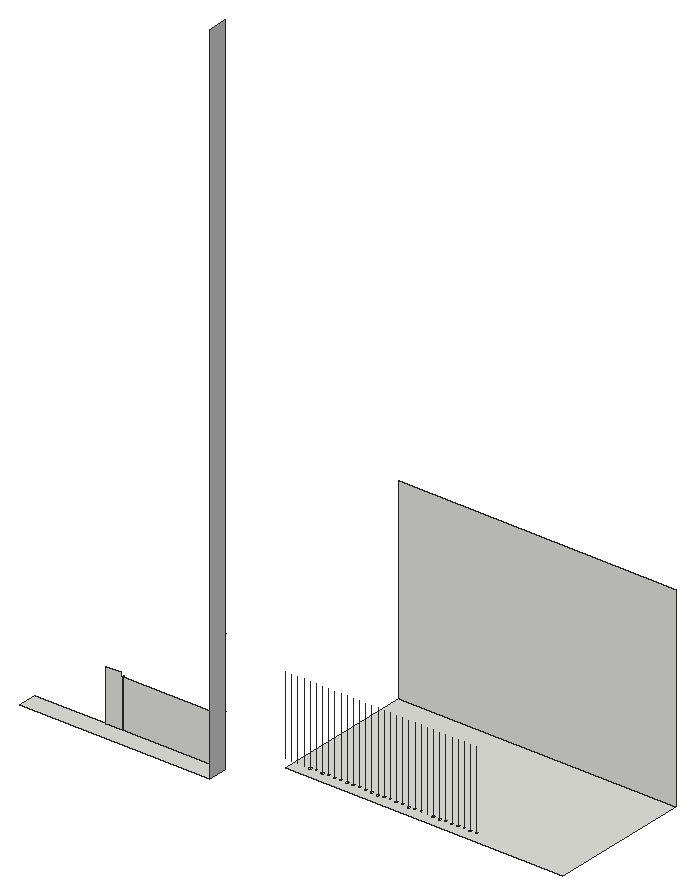
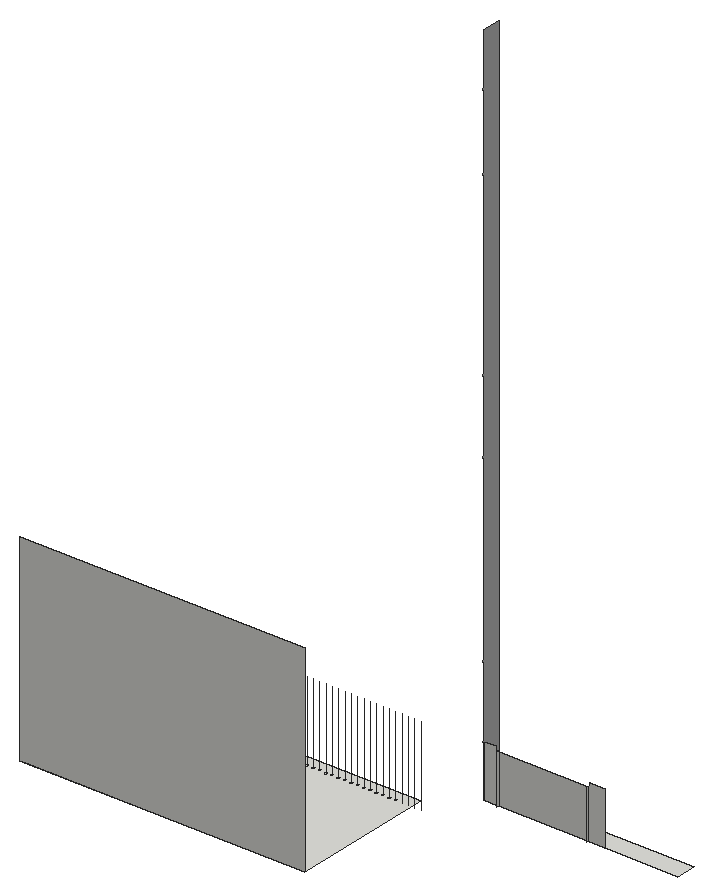
# SketchUp Ruby script. Lengths in inches.
U = 1.inch
M = Sketchup.active_model
def pt(a) = Geom::Point3d.new(a.map { |v| v * U })
def face(e, loops, mat)
  f = e.add_face(loops[0].map { |a| pt(a) })
  loops[1..].each { |l| e.add_face(l.map { |a| pt(a) }).erase! }
  f.material = f.back_material = mat if mat
  f
end
# faces: each face lists its corners as indices into pts; further lists are holes
def faces(e, pts, list, mat = nil) = list.each { |f| face(e, (f[0].is_a?(Array) ? f : [f]).map { |l| l.map { |i| pts[i] } }, mat) }
# xy, xz, yz: faces in a plane at the given z, y or x. An outline is a flat list of corners, or four numbers for a rectangle; further outlines are holes
def ring(l) = l.size == 4 ? [[l[0], l[1]], [l[2], l[1]], [l[2], l[3]], [l[0], l[3]]] : l.each_slice(2).to_a
def flat(e, list, mat, &to3) = list.each { |f| face(e, (f[0].is_a?(Array) ? f : [f]).map { |l| ring(l).map { |u, v| to3.(u, v) } }, mat) }
def xy(e, z, list, mat = nil) = flat(e, list, mat) { |x, y| [x, y, z] }
def xz(e, y, list, mat = nil) = flat(e, list, mat) { |x, z| [x, y, z] }
def yz(e, x, list, mat = nil) = flat(e, list, mat) { |y, z| [x, y, z] }
def lines(e, pts, list) = list.each { |a, b| e.add_line(pt(pts[a]), pt(pts[b])) }
# prism: a flat outline (further loops are holes) pulled along v
def prism(e, loops, v, mat = nil)
  f = face(e, loops, mat); d = Geom::Vector3d.new(v.map { |x| x * U })
  f.pushpull(f.normal.samedirection?(d) ? d.length : -d.length)
end
def box(e, o, s, mat = nil) = prism(e, [[o, [o[0] + s[0], o[1], o[2]], [o[0] + s[0], o[1] + s[1], o[2]], [o[0], o[1] + s[1], o[2]]]], [0, 0, s[2]], mat)
def at(x, y, z, deg = 0) = Geom::Transformation.translation(pt([x, y, z])) * Geom::Transformation.rotation(ORIGIN, Z_AXIS, deg.degrees)
def axes(o, x, y, z) = Geom::Transformation.new([*x, 0, *y, 0, *z, 0, *pt(o).to_a, 1])
def part(name) = M.definitions.add(name)
# library, detail: a bought-in or finely detailed component or shape, given as its bounding box
def library(name, o, s) = part(name).tap { |d| box(d.entities, o, s) }
def detail(e, o, s) = box(e.add_group.entities, o, s)
def put(e, d, t, mat = nil) = e.add_instance(d, t).tap { |i| i.material = mat if mat }
def group(e, t, mat = nil) = e.add_group.tap { |g| g.transformation = t; g.material = mat if mat }.entities
root = M.entities
M.materials.add("Generic\#2").color = [186, 186, 186]
xy(root,409.46,[[96.41,81.125,259.3125,81.125,259.3125,97.25,247.51,97.25,247.51,98.375,247.01,98.375,247.01,97.25,172.16,97.25,172.16,98.375,171.66,98.375,171.66,97.25,96.41,97.25]])
xy(root,409.75,[[409.86,133.41,409.65,133.44,409.45,133.52,409.28,133.65,409.15,133.82,409.07,134.02,409.04,134.23,409.07,134.4375,409.15,134.63,409.28,134.8,409.45,134.93,409.65,135.01,409.86,135.04,410.07,135.01,410.26,134.93,410.43,134.8,410.56,134.63,410.64,134.4375,410.67,134.23,410.64,134.02,410.56,133.82,410.43,133.65,410.26,133.52,410.07,133.44]])
xy(root,409.875,[[[290.4375,124.5,528.75,246],[298.29,133.41,298.08,133.44,297.89,133.52,297.72,133.65,297.59,133.82,297.51,134.02,297.48,134.23,297.51,134.4375,297.59,134.63,297.72,134.8,297.89,134.93,298.08,135.01,298.29,135.04,298.5,135.01,298.7,134.93,298.87,134.8,299,134.63,299.08,134.4375,299.11,134.23,299.08,134.02,299,133.82,298.87,133.65,298.7,133.52,298.5,133.44],[303.61,133.41,303.4,133.44,303.2,133.52,303.03,133.65,302.9,133.82,302.82,134.02,302.79,134.23,302.82,134.4375,302.9,134.63,303.03,134.8,303.2,134.93,303.4,135.01,303.61,135.04,303.82,135.01,304.01,134.93,304.18,134.8,304.31,134.63,304.39,134.4375,304.42,134.23,304.39,134.02,304.31,133.82,304.18,133.65,304.01,133.52,303.82,133.44],[308.92,133.41,308.71,133.44,308.51,133.52,308.34,133.65,308.21,133.82,308.13,134.02,308.11,134.23,308.13,134.4375,308.21,134.63,308.34,134.8,308.51,134.93,308.71,135.01,308.92,135.04,309.13,135.01,309.32,134.93,309.49,134.8,309.62,134.63,309.7,134.4375,309.73,134.23,309.7,134.02,309.62,133.82,309.49,133.65,309.32,133.52,309.13,133.44],[314.23,133.41,314.02,133.44,313.82,133.52,313.66,133.65,313.53,133.82,313.45,134.02,313.42,134.23,313.45,134.4375,313.53,134.63,313.66,134.8,313.82,134.93,314.02,135.01,314.23,135.04,314.44,135.01,314.64,134.93,314.8,134.8,314.93,134.63,315.02,134.4375,315.04,134.23,315.02,134.02,314.93,133.82,314.8,133.65,314.64,133.52,314.44,133.44],[319.54,133.41,319.33,133.44,319.14,133.52,318.97,133.65,318.84,133.82,318.76,134.02,318.73,134.23,318.76,134.4375,318.84,134.63,318.97,134.8,319.14,134.93,319.33,135.01,319.54,135.04,319.75,135.01,319.95,134.93,320.12,134.8,320.25,134.63,320.33,134.4375,320.36,134.23,320.33,134.02,320.25,133.82,320.12,133.65,319.95,133.52,319.75,133.44],[324.86,133.41,324.65,133.44,324.45,133.52,324.28,133.65,324.15,133.82,324.07,134.02,324.04,134.23,324.07,134.4375,324.15,134.63,324.28,134.8,324.45,134.93,324.65,135.01,324.86,135.04,325.07,135.01,325.26,134.93,325.43,134.8,325.56,134.63,325.64,134.4375,325.67,134.23,325.64,134.02,325.56,133.82,325.43,133.65,325.26,133.52,325.07,133.44],[330.17,133.41,329.96,133.44,329.76,133.52,329.59,133.65,329.46,133.82,329.38,134.02,329.36,134.23,329.38,134.4375,329.46,134.63,329.59,134.8,329.76,134.93,329.96,135.01,330.17,135.04,330.38,135.01,330.57,134.93,330.74,134.8,330.87,134.63,330.95,134.4375,330.98,134.23,330.95,134.02,330.87,133.82,330.74,133.65,330.57,133.52,330.38,133.44],[335.48,133.41,335.27,133.44,335.07,133.52,334.91,133.65,334.78,133.82,334.7,134.02,334.67,134.23,334.7,134.4375,334.78,134.63,334.91,134.8,335.07,134.93,335.27,135.01,335.48,135.04,335.69,135.01,335.89,134.93,336.05,134.8,336.18,134.63,336.27,134.4375,336.29,134.23,336.27,134.02,336.18,133.82,336.05,133.65,335.89,133.52,335.69,133.44],[340.79,133.41,340.58,133.44,340.39,133.52,340.22,133.65,340.09,133.82,340.01,134.02,339.98,134.23,340.01,134.4375,340.09,134.63,340.22,134.8,340.39,134.93,340.58,135.01,340.79,135.04,341,135.01,341.2,134.93,341.37,134.8,341.5,134.63,341.58,134.4375,341.61,134.23,341.58,134.02,341.5,133.82,341.37,133.65,341.2,133.52,341,133.44],[346.11,133.41,345.9,133.44,345.7,133.52,345.53,133.65,345.4,133.82,345.32,134.02,345.29,134.23,345.32,134.4375,345.4,134.63,345.53,134.8,345.7,134.93,345.9,135.01,346.11,135.04,346.32,135.01,346.51,134.93,346.68,134.8,346.81,134.63,346.89,134.4375,346.92,134.23,346.89,134.02,346.81,133.82,346.68,133.65,346.51,133.52,346.32,133.44],[351.42,133.41,351.21,133.44,351.01,133.52,350.84,133.65,350.71,133.82,350.63,134.02,350.61,134.23,350.63,134.4375,350.71,134.63,350.84,134.8,351.01,134.93,351.21,135.01,351.42,135.04,351.63,135.01,351.82,134.93,351.99,134.8,352.12,134.63,352.2,134.4375,352.23,134.23,352.2,134.02,352.12,133.82,351.99,133.65,351.82,133.52,351.63,133.44],[356.73,133.41,356.52,133.44,356.32,133.52,356.16,133.65,356.03,133.82,355.95,134.02,355.92,134.23,355.95,134.4375,356.03,134.63,356.16,134.8,356.32,134.93,356.52,135.01,356.73,135.04,356.94,135.01,357.14,134.93,357.3,134.8,357.43,134.63,357.52,134.4375,357.54,134.23,357.52,134.02,357.43,133.82,357.3,133.65,357.14,133.52,356.94,133.44],[362.04,133.41,361.83,133.44,361.64,133.52,361.47,133.65,361.34,133.82,361.26,134.02,361.23,134.23,361.26,134.4375,361.34,134.63,361.47,134.8,361.64,134.93,361.83,135.01,362.04,135.04,362.25,135.01,362.45,134.93,362.62,134.8,362.75,134.63,362.83,134.4375,362.86,134.23,362.83,134.02,362.75,133.82,362.62,133.65,362.45,133.52,362.25,133.44],[367.36,133.41,367.15,133.44,366.95,133.52,366.78,133.65,366.65,133.82,366.57,134.02,366.54,134.23,366.57,134.4375,366.65,134.63,366.78,134.8,366.95,134.93,367.15,135.01,367.36,135.04,367.57,135.01,367.76,134.93,367.93,134.8,368.06,134.63,368.14,134.4375,368.17,134.23,368.14,134.02,368.06,133.82,367.93,133.65,367.76,133.52,367.57,133.44],[372.67,133.41,372.46,133.44,372.26,133.52,372.09,133.65,371.96,133.82,371.88,134.02,371.86,134.23,371.88,134.4375,371.96,134.63,372.09,134.8,372.26,134.93,372.46,135.01,372.67,135.04,372.88,135.01,373.07,134.93,373.24,134.8,373.37,134.63,373.45,134.4375,373.48,134.23,373.45,134.02,373.37,133.82,373.24,133.65,373.07,133.52,372.88,133.44],[377.98,133.41,377.77,133.44,377.57,133.52,377.41,133.65,377.28,133.82,377.2,134.02,377.17,134.23,377.2,134.4375,377.28,134.63,377.41,134.8,377.57,134.93,377.77,135.01,377.98,135.04,378.19,135.01,378.39,134.93,378.55,134.8,378.68,134.63,378.77,134.4375,378.79,134.23,378.77,134.02,378.68,133.82,378.55,133.65,378.39,133.52,378.19,133.44],[383.29,133.41,383.08,133.44,382.89,133.52,382.72,133.65,382.59,133.82,382.51,134.02,382.48,134.23,382.51,134.4375,382.59,134.63,382.72,134.8,382.89,134.93,383.08,135.01,383.29,135.04,383.5,135.01,383.7,134.93,383.87,134.8,384,134.63,384.08,134.4375,384.11,134.23,384.08,134.02,384,133.82,383.87,133.65,383.7,133.52,383.5,133.44],[388.61,133.41,388.4,133.44,388.2,133.52,388.03,133.65,387.9,133.82,387.82,134.02,387.79,134.23,387.82,134.4375,387.9,134.63,388.03,134.8,388.2,134.93,388.4,135.01,388.61,135.04,388.82,135.01,389.01,134.93,389.18,134.8,389.31,134.63,389.39,134.4375,389.42,134.23,389.39,134.02,389.31,133.82,389.18,133.65,389.01,133.52,388.82,133.44],[393.92,133.41,393.71,133.44,393.51,133.52,393.34,133.65,393.21,133.82,393.13,134.02,393.11,134.23,393.13,134.4375,393.21,134.63,393.34,134.8,393.51,134.93,393.71,135.01,393.92,135.04,394.13,135.01,394.32,134.93,394.49,134.8,394.62,134.63,394.7,134.4375,394.73,134.23,394.7,134.02,394.62,133.82,394.49,133.65,394.32,133.52,394.13,133.44],[399.23,133.41,399.02,133.44,398.82,133.52,398.66,133.65,398.53,133.82,398.45,134.02,398.42,134.23,398.45,134.4375,398.53,134.63,398.66,134.8,398.82,134.93,399.02,135.01,399.23,135.04,399.44,135.01,399.64,134.93,399.8,134.8,399.93,134.63,400.02,134.4375,400.04,134.23,400.02,134.02,399.93,133.82,399.8,133.65,399.64,133.52,399.44,133.44],[404.54,133.41,404.33,133.44,404.14,133.52,403.97,133.65,403.84,133.82,403.76,134.02,403.73,134.23,403.76,134.4375,403.84,134.63,403.97,134.8,404.14,134.93,404.33,135.01,404.54,135.04,404.75,135.01,404.95,134.93,405.12,134.8,405.25,134.63,405.33,134.4375,405.36,134.23,405.33,134.02,405.25,133.82,405.12,133.65,404.95,133.52,404.75,133.44],[409.86,133.41,409.65,133.44,409.45,133.52,409.28,133.65,409.15,133.82,409.07,134.02,409.04,134.23,409.07,134.4375,409.15,134.63,409.28,134.8,409.45,134.93,409.65,135.01,409.86,135.04,410.07,135.01,410.26,134.93,410.43,134.8,410.56,134.63,410.64,134.4375,410.67,134.23,410.64,134.02,410.56,133.82,410.43,133.65,410.26,133.52,410.07,133.44],[415.17,133.41,414.96,133.44,414.76,133.52,414.59,133.65,414.46,133.82,414.38,134.02,414.36,134.23,414.38,134.4375,414.46,134.63,414.59,134.8,414.76,134.93,414.96,135.01,415.17,135.04,415.38,135.01,415.57,134.93,415.74,134.8,415.87,134.63,415.95,134.4375,415.98,134.23,415.95,134.02,415.87,133.82,415.74,133.65,415.57,133.52,415.38,133.44],[420.48,133.41,420.27,133.44,420.07,133.52,419.91,133.65,419.78,133.82,419.7,134.02,419.67,134.23,419.7,134.4375,419.78,134.63,419.91,134.8,420.07,134.93,420.27,135.01,420.48,135.04,420.69,135.01,420.89,134.93,421.05,134.8,421.18,134.63,421.27,134.4375,421.29,134.23,421.27,134.02,421.18,133.82,421.05,133.65,420.89,133.52,420.69,133.44],[425.79,133.41,425.58,133.44,425.39,133.52,425.22,133.65,425.09,133.82,425.01,134.02,424.98,134.23,425.01,134.4375,425.09,134.63,425.22,134.8,425.39,134.93,425.58,135.01,425.79,135.04,426,135.01,426.2,134.93,426.37,134.8,426.5,134.63,426.58,134.4375,426.61,134.23,426.58,134.02,426.5,133.82,426.37,133.65,426.2,133.52,426,133.44],[431.11,133.41,430.9,133.44,430.7,133.52,430.53,133.65,430.4,133.82,430.32,134.02,430.29,134.23,430.32,134.4375,430.4,134.63,430.53,134.8,430.7,134.93,430.9,135.01,431.11,135.04,431.32,135.01,431.51,134.93,431.68,134.8,431.81,134.63,431.89,134.4375,431.92,134.23,431.89,134.02,431.81,133.82,431.68,133.65,431.51,133.52,431.32,133.44],[436.42,133.41,436.21,133.44,436.01,133.52,435.84,133.65,435.71,133.82,435.63,134.02,435.61,134.23,435.63,134.4375,435.71,134.63,435.84,134.8,436.01,134.93,436.21,135.01,436.42,135.04,436.63,135.01,436.82,134.93,436.99,134.8,437.12,134.63,437.2,134.4375,437.23,134.23,437.2,134.02,437.12,133.82,436.99,133.65,436.82,133.52,436.63,133.44],[441.73,133.41,441.52,133.44,441.32,133.52,441.16,133.65,441.03,133.82,440.95,134.02,440.92,134.23,440.95,134.4375,441.03,134.63,441.16,134.8,441.32,134.93,441.52,135.01,441.73,135.04,441.94,135.01,442.14,134.93,442.3,134.8,442.43,134.63,442.52,134.4375,442.54,134.23,442.52,134.02,442.43,133.82,442.3,133.65,442.14,133.52,441.94,133.44],[447.04,133.41,446.83,133.44,446.64,133.52,446.47,133.65,446.34,133.82,446.26,134.02,446.23,134.23,446.26,134.4375,446.34,134.63,446.47,134.8,446.64,134.93,446.83,135.01,447.04,135.04,447.25,135.01,447.45,134.93,447.62,134.8,447.75,134.63,447.83,134.4375,447.86,134.23,447.83,134.02,447.75,133.82,447.62,133.65,447.45,133.52,447.25,133.44],[452.36,133.41,452.15,133.44,451.95,133.52,451.78,133.65,451.65,133.82,451.57,134.02,451.54,134.23,451.57,134.4375,451.65,134.63,451.78,134.8,451.95,134.93,452.15,135.01,452.36,135.04,452.57,135.01,452.76,134.93,452.93,134.8,453.06,134.63,453.14,134.4375,453.17,134.23,453.14,134.02,453.06,133.82,452.93,133.65,452.76,133.52,452.57,133.44],[457.67,133.41,457.46,133.44,457.26,133.52,457.09,133.65,456.96,133.82,456.88,134.02,456.86,134.23,456.88,134.4375,456.96,134.63,457.09,134.8,457.26,134.93,457.46,135.01,457.67,135.04,457.88,135.01,458.07,134.93,458.24,134.8,458.37,134.63,458.45,134.4375,458.48,134.23,458.45,134.02,458.37,133.82,458.24,133.65,458.07,133.52,457.88,133.44],[462.92,133.41,462.71,133.44,462.51,133.52,462.34,133.65,462.21,133.82,462.13,134.02,462.11,134.23,462.13,134.4375,462.21,134.63,462.34,134.8,462.51,134.93,462.71,135.01,462.92,135.04,463.13,135.01,463.32,134.93,463.49,134.8,463.62,134.63,463.7,134.4375,463.73,134.23,463.7,134.02,463.62,133.82,463.49,133.65,463.32,133.52,463.13,133.44],[468.17,133.41,467.96,133.44,467.76,133.52,467.59,133.65,467.46,133.82,467.38,134.02,467.36,134.23,467.38,134.4375,467.46,134.63,467.59,134.8,467.76,134.93,467.96,135.01,468.17,135.04,468.38,135.01,468.57,134.93,468.74,134.8,468.87,134.63,468.95,134.4375,468.98,134.23,468.95,134.02,468.87,133.82,468.74,133.65,468.57,133.52,468.38,133.44],[473.42,133.41,473.21,133.44,473.01,133.52,472.84,133.65,472.71,133.82,472.63,134.02,472.61,134.23,472.63,134.4375,472.71,134.63,472.84,134.8,473.01,134.93,473.21,135.01,473.42,135.04,473.63,135.01,473.82,134.93,473.99,134.8,474.12,134.63,474.2,134.4375,474.23,134.23,474.2,134.02,474.12,133.82,473.99,133.65,473.82,133.52,473.63,133.44],[478.67,133.41,478.46,133.44,478.26,133.52,478.09,133.65,477.96,133.82,477.88,134.02,477.86,134.23,477.88,134.4375,477.96,134.63,478.09,134.8,478.26,134.93,478.46,135.01,478.67,135.04,478.88,135.01,479.07,134.93,479.24,134.8,479.37,134.63,479.45,134.4375,479.48,134.23,479.45,134.02,479.37,133.82,479.24,133.65,479.07,133.52,478.88,133.44],[483.92,133.41,483.71,133.44,483.51,133.52,483.34,133.65,483.21,133.82,483.13,134.02,483.11,134.23,483.13,134.4375,483.21,134.63,483.34,134.8,483.51,134.93,483.71,135.01,483.92,135.04,484.13,135.01,484.32,134.93,484.49,134.8,484.62,134.63,484.7,134.4375,484.73,134.23,484.7,134.02,484.62,133.82,484.49,133.65,484.32,133.52,484.13,133.44],[489.54,133.41,489.33,133.44,489.14,133.52,488.97,133.65,488.84,133.82,488.76,134.02,488.73,134.23,488.76,134.4375,488.84,134.63,488.97,134.8,489.14,134.93,489.33,135.01,489.54,135.04,489.75,135.01,489.95,134.93,490.12,134.8,490.25,134.63,490.33,134.4375,490.36,134.23,490.33,134.02,490.25,133.82,490.12,133.65,489.95,133.52,489.75,133.44],[494.86,133.41,494.65,133.44,494.45,133.52,494.28,133.65,494.15,133.82,494.07,134.02,494.04,134.23,494.07,134.4375,494.15,134.63,494.28,134.8,494.45,134.93,494.65,135.01,494.86,135.04,495.07,135.01,495.26,134.93,495.43,134.8,495.56,134.63,495.64,134.4375,495.67,134.23,495.64,134.02,495.56,133.82,495.43,133.65,495.26,133.52,495.07,133.44],[500.17,133.41,499.96,133.44,499.76,133.52,499.59,133.65,499.46,133.82,499.38,134.02,499.36,134.23,499.38,134.4375,499.46,134.63,499.59,134.8,499.76,134.93,499.96,135.01,500.17,135.04,500.38,135.01,500.57,134.93,500.74,134.8,500.87,134.63,500.95,134.4375,500.98,134.23,500.95,134.02,500.87,133.82,500.74,133.65,500.57,133.52,500.38,133.44],[505.42,133.41,505.21,133.44,505.01,133.52,504.84,133.65,504.71,133.82,504.63,134.02,504.61,134.23,504.63,134.4375,504.71,134.63,504.84,134.8,505.01,134.93,505.21,135.01,505.42,135.04,505.63,135.01,505.82,134.93,505.99,134.8,506.12,134.63,506.2,134.4375,506.23,134.23,506.2,134.02,506.12,133.82,505.99,133.65,505.82,133.52,505.63,133.44],[510.67,133.41,510.46,133.44,510.26,133.52,510.09,133.65,509.96,133.82,509.88,134.02,509.86,134.23,509.88,134.4375,509.96,134.63,510.09,134.8,510.26,134.93,510.46,135.01,510.67,135.04,510.88,135.01,511.07,134.93,511.24,134.8,511.37,134.63,511.45,134.4375,511.48,134.23,511.45,134.02,511.37,133.82,511.24,133.65,511.07,133.52,510.88,133.44],[515.92,133.41,515.71,133.44,515.51,133.52,515.34,133.65,515.21,133.82,515.13,134.02,515.11,134.23,515.13,134.4375,515.21,134.63,515.34,134.8,515.51,134.93,515.71,135.01,515.92,135.04,516.13,135.01,516.32,134.93,516.49,134.8,516.62,134.63,516.7,134.4375,516.73,134.23,516.7,134.02,516.62,133.82,516.49,133.65,516.32,133.52,516.13,133.44],[521.23,133.41,521.02,133.44,520.82,133.52,520.66,133.65,520.53,133.82,520.45,134.02,520.42,134.23,520.45,134.4375,520.53,134.63,520.66,134.8,520.82,134.93,521.02,135.01,521.23,135.04,521.44,135.01,521.64,134.93,521.8,134.8,521.93,134.63,522.02,134.4375,522.04,134.23,522.02,134.02,521.93,133.82,521.8,133.65,521.64,133.52,521.44,133.44]],[303.61,133.41,303.4,133.44,303.2,133.52,303.03,133.65,302.9,133.82,302.82,134.02,302.79,134.23,302.82,134.4375,302.9,134.63,303.03,134.8,303.2,134.93,303.4,135.01,303.61,135.04,303.82,135.01,304.01,134.93,304.18,134.8,304.31,134.63,304.39,134.4375,304.42,134.23,304.39,134.02,304.31,133.82,304.18,133.65,304.01,133.52,303.82,133.44],[308.92,133.41,308.71,133.44,308.51,133.52,308.34,133.65,308.21,133.82,308.13,134.02,308.11,134.23,308.13,134.4375,308.21,134.63,308.34,134.8,308.51,134.93,308.71,135.01,308.92,135.04,309.13,135.01,309.32,134.93,309.49,134.8,309.62,134.63,309.7,134.4375,309.73,134.23,309.7,134.02,309.62,133.82,309.49,133.65,309.32,133.52,309.13,133.44],[314.23,133.41,314.02,133.44,313.82,133.52,313.66,133.65,313.53,133.82,313.45,134.02,313.42,134.23,313.45,134.4375,313.53,134.63,313.66,134.8,313.82,134.93,314.02,135.01,314.23,135.04,314.44,135.01,314.64,134.93,314.8,134.8,314.93,134.63,315.02,134.4375,315.04,134.23,315.02,134.02,314.93,133.82,314.8,133.65,314.64,133.52,314.44,133.44],[319.54,133.41,319.33,133.44,319.14,133.52,318.97,133.65,318.84,133.82,318.76,134.02,318.73,134.23,318.76,134.4375,318.84,134.63,318.97,134.8,319.14,134.93,319.33,135.01,319.54,135.04,319.75,135.01,319.95,134.93,320.12,134.8,320.25,134.63,320.33,134.4375,320.36,134.23,320.33,134.02,320.25,133.82,320.12,133.65,319.95,133.52,319.75,133.44],
  [324.86,133.41,324.65,133.44,324.45,133.52,324.28,133.65,324.15,133.82,324.07,134.02,324.04,134.23,324.07,134.4375,324.15,134.63,324.28,134.8,324.45,134.93,324.65,135.01,324.86,135.04,325.07,135.01,325.26,134.93,325.43,134.8,325.56,134.63,325.64,134.4375,325.67,134.23,325.64,134.02,325.56,133.82,325.43,133.65,325.26,133.52,325.07,133.44],[330.17,133.41,329.96,133.44,329.76,133.52,329.59,133.65,329.46,133.82,329.38,134.02,329.36,134.23,329.38,134.4375,329.46,134.63,329.59,134.8,329.76,134.93,329.96,135.01,330.17,135.04,330.38,135.01,330.57,134.93,330.74,134.8,330.87,134.63,330.95,134.4375,330.98,134.23,330.95,134.02,330.87,133.82,330.74,133.65,330.57,133.52,330.38,133.44],[335.48,133.41,335.27,133.44,335.07,133.52,334.91,133.65,334.78,133.82,334.7,134.02,334.67,134.23,334.7,134.4375,334.78,134.63,334.91,134.8,335.07,134.93,335.27,135.01,335.48,135.04,335.69,135.01,335.89,134.93,336.05,134.8,336.18,134.63,336.27,134.4375,336.29,134.23,336.27,134.02,336.18,133.82,336.05,133.65,335.89,133.52,335.69,133.44],[340.79,133.41,340.58,133.44,340.39,133.52,340.22,133.65,340.09,133.82,340.01,134.02,339.98,134.23,340.01,134.4375,340.09,134.63,340.22,134.8,340.39,134.93,340.58,135.01,340.79,135.04,341,135.01,341.2,134.93,341.37,134.8,341.5,134.63,341.58,134.4375,341.61,134.23,341.58,134.02,341.5,133.82,341.37,133.65,341.2,133.52,341,133.44],[346.11,133.41,345.9,133.44,345.7,133.52,345.53,133.65,345.4,133.82,345.32,134.02,345.29,134.23,345.32,134.4375,345.4,134.63,345.53,134.8,345.7,134.93,345.9,135.01,346.11,135.04,346.32,135.01,346.51,134.93,346.68,134.8,346.81,134.63,346.89,134.4375,346.92,134.23,346.89,134.02,346.81,133.82,346.68,133.65,346.51,133.52,346.32,133.44],
  [351.42,133.41,351.21,133.44,351.01,133.52,350.84,133.65,350.71,133.82,350.63,134.02,350.61,134.23,350.63,134.4375,350.71,134.63,350.84,134.8,351.01,134.93,351.21,135.01,351.42,135.04,351.63,135.01,351.82,134.93,351.99,134.8,352.12,134.63,352.2,134.4375,352.23,134.23,352.2,134.02,352.12,133.82,351.99,133.65,351.82,133.52,351.63,133.44],[356.73,133.41,356.52,133.44,356.32,133.52,356.16,133.65,356.03,133.82,355.95,134.02,355.92,134.23,355.95,134.4375,356.03,134.63,356.16,134.8,356.32,134.93,356.52,135.01,356.73,135.04,356.94,135.01,357.14,134.93,357.3,134.8,357.43,134.63,357.52,134.4375,357.54,134.23,357.52,134.02,357.43,133.82,357.3,133.65,357.14,133.52,356.94,133.44],[362.04,133.41,361.83,133.44,361.64,133.52,361.47,133.65,361.34,133.82,361.26,134.02,361.23,134.23,361.26,134.4375,361.34,134.63,361.47,134.8,361.64,134.93,361.83,135.01,362.04,135.04,362.25,135.01,362.45,134.93,362.62,134.8,362.75,134.63,362.83,134.4375,362.86,134.23,362.83,134.02,362.75,133.82,362.62,133.65,362.45,133.52,362.25,133.44],[367.36,133.41,367.15,133.44,366.95,133.52,366.78,133.65,366.65,133.82,366.57,134.02,366.54,134.23,366.57,134.4375,366.65,134.63,366.78,134.8,366.95,134.93,367.15,135.01,367.36,135.04,367.57,135.01,367.76,134.93,367.93,134.8,368.06,134.63,368.14,134.4375,368.17,134.23,368.14,134.02,368.06,133.82,367.93,133.65,367.76,133.52,367.57,133.44],[372.67,133.41,372.46,133.44,372.26,133.52,372.09,133.65,371.96,133.82,371.88,134.02,371.86,134.23,371.88,134.4375,371.96,134.63,372.09,134.8,372.26,134.93,372.46,135.01,372.67,135.04,372.88,135.01,373.07,134.93,373.24,134.8,373.37,134.63,373.45,134.4375,373.48,134.23,373.45,134.02,373.37,133.82,373.24,133.65,373.07,133.52,372.88,133.44],
  [377.98,133.41,377.77,133.44,377.57,133.52,377.41,133.65,377.28,133.82,377.2,134.02,377.17,134.23,377.2,134.4375,377.28,134.63,377.41,134.8,377.57,134.93,377.77,135.01,377.98,135.04,378.19,135.01,378.39,134.93,378.55,134.8,378.68,134.63,378.77,134.4375,378.79,134.23,378.77,134.02,378.68,133.82,378.55,133.65,378.39,133.52,378.19,133.44],[383.29,133.41,383.08,133.44,382.89,133.52,382.72,133.65,382.59,133.82,382.51,134.02,382.48,134.23,382.51,134.4375,382.59,134.63,382.72,134.8,382.89,134.93,383.08,135.01,383.29,135.04,383.5,135.01,383.7,134.93,383.87,134.8,384,134.63,384.08,134.4375,384.11,134.23,384.08,134.02,384,133.82,383.87,133.65,383.7,133.52,383.5,133.44],[388.61,133.41,388.4,133.44,388.2,133.52,388.03,133.65,387.9,133.82,387.82,134.02,387.79,134.23,387.82,134.4375,387.9,134.63,388.03,134.8,388.2,134.93,388.4,135.01,388.61,135.04,388.82,135.01,389.01,134.93,389.18,134.8,389.31,134.63,389.39,134.4375,389.42,134.23,389.39,134.02,389.31,133.82,389.18,133.65,389.01,133.52,388.82,133.44],[393.92,133.41,393.71,133.44,393.51,133.52,393.34,133.65,393.21,133.82,393.13,134.02,393.11,134.23,393.13,134.4375,393.21,134.63,393.34,134.8,393.51,134.93,393.71,135.01,393.92,135.04,394.13,135.01,394.32,134.93,394.49,134.8,394.62,134.63,394.7,134.4375,394.73,134.23,394.7,134.02,394.62,133.82,394.49,133.65,394.32,133.52,394.13,133.44],[399.23,133.41,399.02,133.44,398.82,133.52,398.66,133.65,398.53,133.82,398.45,134.02,398.42,134.23,398.45,134.4375,398.53,134.63,398.66,134.8,398.82,134.93,399.02,135.01,399.23,135.04,399.44,135.01,399.64,134.93,399.8,134.8,399.93,134.63,400.02,134.4375,400.04,134.23,400.02,134.02,399.93,133.82,399.8,133.65,399.64,133.52,399.44,133.44],
  [409.86,133.41,409.65,133.44,409.45,133.52,409.28,133.65,409.15,133.82,409.07,134.02,409.04,134.23,409.07,134.4375,409.15,134.63,409.28,134.8,409.45,134.93,409.65,135.01,409.86,135.04,410.07,135.01,410.26,134.93,410.43,134.8,410.56,134.63,410.64,134.4375,410.67,134.23,410.64,134.02,410.56,133.82,410.43,133.65,410.26,133.52,410.07,133.44],[415.17,133.41,414.96,133.44,414.76,133.52,414.59,133.65,414.46,133.82,414.38,134.02,414.36,134.23,414.38,134.4375,414.46,134.63,414.59,134.8,414.76,134.93,414.96,135.01,415.17,135.04,415.38,135.01,415.57,134.93,415.74,134.8,415.87,134.63,415.95,134.4375,415.98,134.23,415.95,134.02,415.87,133.82,415.74,133.65,415.57,133.52,415.38,133.44],[420.48,133.41,420.27,133.44,420.07,133.52,419.91,133.65,419.78,133.82,419.7,134.02,419.67,134.23,419.7,134.4375,419.78,134.63,419.91,134.8,420.07,134.93,420.27,135.01,420.48,135.04,420.69,135.01,420.89,134.93,421.05,134.8,421.18,134.63,421.27,134.4375,421.29,134.23,421.27,134.02,421.18,133.82,421.05,133.65,420.89,133.52,420.69,133.44],[425.79,133.41,425.58,133.44,425.39,133.52,425.22,133.65,425.09,133.82,425.01,134.02,424.98,134.23,425.01,134.4375,425.09,134.63,425.22,134.8,425.39,134.93,425.58,135.01,425.79,135.04,426,135.01,426.2,134.93,426.37,134.8,426.5,134.63,426.58,134.4375,426.61,134.23,426.58,134.02,426.5,133.82,426.37,133.65,426.2,133.52,426,133.44],[431.11,133.41,430.9,133.44,430.7,133.52,430.53,133.65,430.4,133.82,430.32,134.02,430.29,134.23,430.32,134.4375,430.4,134.63,430.53,134.8,430.7,134.93,430.9,135.01,431.11,135.04,431.32,135.01,431.51,134.93,431.68,134.8,431.81,134.63,431.89,134.4375,431.92,134.23,431.89,134.02,431.81,133.82,431.68,133.65,431.51,133.52,431.32,133.44],
  [436.42,133.41,436.21,133.44,436.01,133.52,435.84,133.65,435.71,133.82,435.63,134.02,435.61,134.23,435.63,134.4375,435.71,134.63,435.84,134.8,436.01,134.93,436.21,135.01,436.42,135.04,436.63,135.01,436.82,134.93,436.99,134.8,437.12,134.63,437.2,134.4375,437.23,134.23,437.2,134.02,437.12,133.82,436.99,133.65,436.82,133.52,436.63,133.44],[441.73,133.41,441.52,133.44,441.32,133.52,441.16,133.65,441.03,133.82,440.95,134.02,440.92,134.23,440.95,134.4375,441.03,134.63,441.16,134.8,441.32,134.93,441.52,135.01,441.73,135.04,441.94,135.01,442.14,134.93,442.3,134.8,442.43,134.63,442.52,134.4375,442.54,134.23,442.52,134.02,442.43,133.82,442.3,133.65,442.14,133.52,441.94,133.44],[447.04,133.41,446.83,133.44,446.64,133.52,446.47,133.65,446.34,133.82,446.26,134.02,446.23,134.23,446.26,134.4375,446.34,134.63,446.47,134.8,446.64,134.93,446.83,135.01,447.04,135.04,447.25,135.01,447.45,134.93,447.62,134.8,447.75,134.63,447.83,134.4375,447.86,134.23,447.83,134.02,447.75,133.82,447.62,133.65,447.45,133.52,447.25,133.44]])
xz(root,97.25,[[157.47,409.46,171.66,409.46,171.66,450.375,170.35,450.375,170.35,453.4375,157.47,453.4375],[172.16,409.46,247.01,450.375],[247.51,409.46,259.3125,409.46,259.3125,453.4375,249.19,453.4375,249.19,450.375,247.51,450.375]])
xz(root,98.375,[[171.66,409.46,172.16,450.375],[247.01,409.46,247.51,450.375]])
xz(root,246,[[290.4375,409.875,528.75,577.875]])
yz(root,171.66,[[97.25,409.46,98.375,450.375]])
yz(root,172.16,[[97.25,409.46,98.375,450.375]])
yz(root,247.01,[[97.25,409.46,98.375,450.375]])
yz(root,247.51,[[97.25,409.46,98.375,450.375]])
yz(root,259.3125,[[81.125,409.46,81.125,987.75,97.25,987.75,97.25,943.6875,98,943.6875,98,943.1875,97.25,943.1875,97.25,880,98,880,98,879.5,97.25,879.5,97.25,728.75,98,728.75,98,728.25,97.25,728.25,97.25,667.5,98,667.5,98,667,97.25,667,97.25,514.1875,98.375,514.1875,98.375,513.6875,97.25,513.6875,97.25,453.9375,98.375,453.9375,98.375,453.4375,97.25,453.4375,97.25,409.46]],"Generic\#2")
p = [[409.65,133.44,409.875],[409.45,133.52,409.875],[409.45,133.52,409.75],[409.65,133.44,409.75],[409.86,133.41,409.875],[409.86,133.41,409.75],
  [410.07,133.44,409.875],[410.07,133.44,409.75],[410.26,133.52,409.875],[410.26,133.52,409.75],[409.28,133.65,409.875],[409.28,133.65,409.75],
  [410.43,133.65,409.875],[410.43,133.65,409.75],[409.15,133.82,409.875],[409.15,133.82,409.75],[410.56,133.82,409.875],[410.56,133.82,409.75],
  [409.07,134.02,409.875],[409.07,134.02,409.75],[410.64,134.02,409.875],[410.64,134.02,409.75],[409.04,134.23,409.875],[409.04,134.23,409.75],
  [410.67,134.23,409.875],[410.67,134.23,409.75],[409.07,134.4375,409.875],[409.07,134.4375,409.75],[410.64,134.4375,409.875],[410.64,134.4375,409.75],
  [409.15,134.63,409.875],[409.15,134.63,409.75],[410.56,134.63,409.875],[410.56,134.63,409.75],[409.28,134.8,409.875],[409.28,134.8,409.75],
  [410.43,134.8,409.875],[410.43,134.8,409.75],[409.45,134.93,409.875],[409.45,134.93,409.75],[410.26,134.93,409.875],[410.26,134.93,409.75],
  [409.65,135.01,409.875],[409.65,135.01,409.75],[410.07,135.01,409.875],[410.07,135.01,409.75],[409.86,135.04,409.875],[409.86,135.04,409.75],
  [447.01,134.22,477.08],[447.01,134.22,409.875],[441.7,134.22,477.08],[441.7,134.22,409.875],[436.39,134.22,477.08],[436.39,134.22,409.875],
  [431.07,134.22,477.08],[431.07,134.22,409.875],[425.76,134.22,477.08],[425.76,134.22,409.875],[420.45,134.22,477.08],[420.45,134.22,409.875],
  [415.14,134.22,477.08],[415.14,134.22,409.875],[409.82,134.22,477.08],[409.82,134.22,409.875],[404.51,134.22,477.08],[404.51,134.22,409.875],
  [399.2,134.22,477.08],[399.2,134.22,409.875],[393.89,134.22,477.08],[393.89,134.22,409.875],[388.57,134.22,477.08],[388.57,134.22,409.875],
  [383.26,134.22,477.08],[383.26,134.22,409.875],[377.95,134.22,477.08],[377.95,134.22,409.875],[372.64,134.22,477.08],[372.64,134.22,409.875],
  [367.32,134.22,477.08],[367.32,134.22,409.875],[362.01,134.22,477.08],[362.01,134.22,409.875],[356.7,134.22,477.08],[356.7,134.22,409.875],
  [351.39,134.22,477.08],[351.39,134.22,409.875],[346.07,134.22,477.08],[346.07,134.22,409.875],[340.76,134.22,477.08],[340.76,134.22,409.875],
  [335.45,134.22,477.08],[335.45,134.22,409.875],[330.14,134.22,477.08],[330.14,134.22,409.875],[324.82,134.22,477.08],[324.82,134.22,409.875],
  [319.51,134.22,477.08],[319.51,134.22,409.875],[314.2,134.22,477.08],[314.2,134.22,409.875],[308.89,134.22,477.08],[308.89,134.22,409.875],
  [303.57,134.22,477.08],[303.57,134.22,409.875],[298.26,134.22,477.08],[298.26,134.22,409.875],[292.95,134.22,477.08],[292.95,134.22,409.875],
  [287.64,134.22,477.08],[287.64,134.22,409.875],[282.32,134.22,477.08],[282.32,134.22,409.875]]
faces(root,p,[[0,1,2,3],[4,0,3,5],[6,4,5,7],[8,6,7,9],[1,10,11,2],[12,8,9,13],[10,14,15,11],[16,12,13,17],
  [14,18,19,15],[20,16,17,21],[18,22,23,19],[24,20,21,25],[22,26,27,23],[28,24,25,29],[26,30,31,27],[32,28,29,33],
  [30,34,35,31],[36,32,33,37],[34,38,39,35],[40,36,37,41],[38,42,43,39],[44,40,41,45],[42,46,47,43],[46,44,45,47]])
lines(root,p,[[48,49],[50,51],[52,53],[54,55],[56,57],[58,59],[60,61],[62,63],[64,65],[66,67],[68,69],[70,71],
  [72,73],[74,75],[76,77],[78,79],[80,81],[82,83],[84,85],[86,87],[88,89],[90,91],[92,93],[94,95],
  [96,97],[98,99],[100,101],[102,103],[104,105],[106,107],[108,109],[110,111]])
